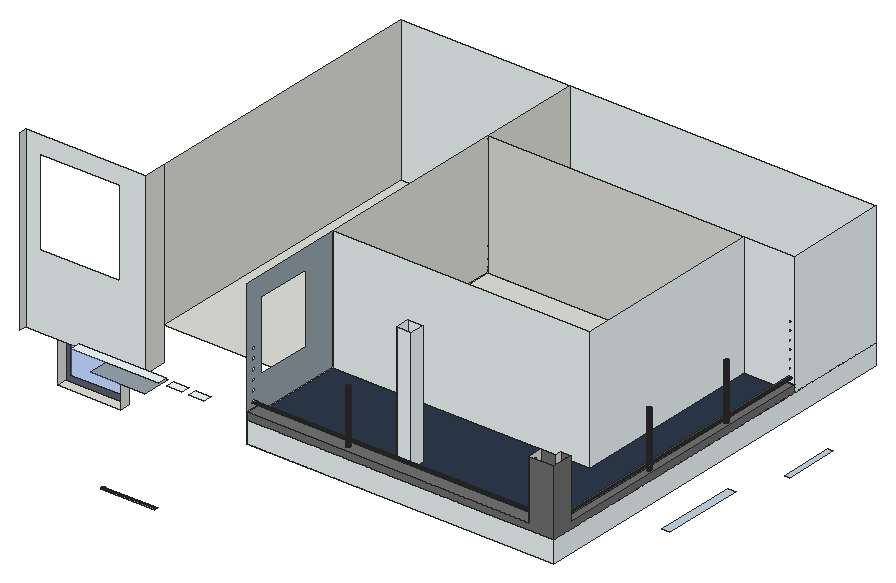
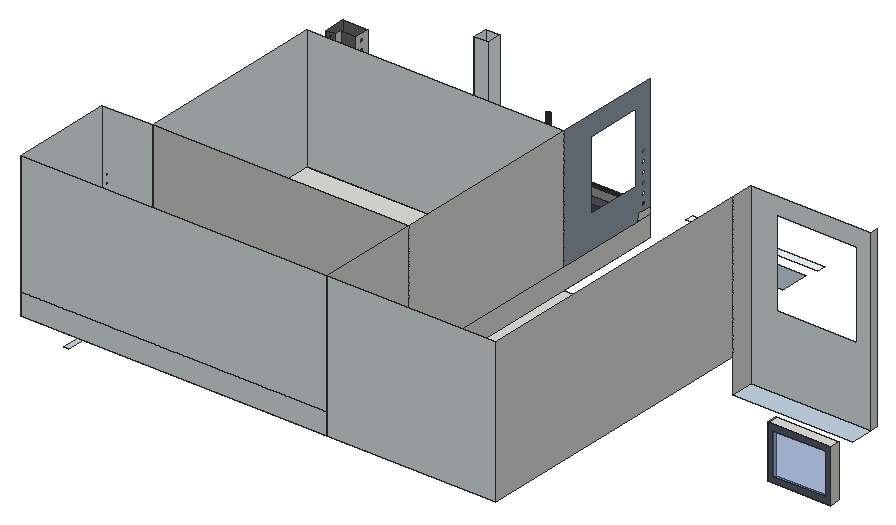
# SketchUp Ruby script. Lengths in inches.
U = 1.inch
M = Sketchup.active_model
def pt(a) = Geom::Point3d.new(a.map { |v| v * U })
def face(e, loops, mat)
  f = e.add_face(loops[0].map { |a| pt(a) })
  loops[1..].each { |l| e.add_face(l.map { |a| pt(a) }).erase! }
  f.material = f.back_material = mat if mat
  f
end
# faces: each face lists its corners as indices into pts; further lists are holes
def faces(e, pts, list, mat = nil) = list.each { |f| face(e, (f[0].is_a?(Array) ? f : [f]).map { |l| l.map { |i| pts[i] } }, mat) }
# xy, xz, yz: faces in a plane at the given z, y or x. An outline is a flat list of corners, or four numbers for a rectangle; further outlines are holes
def ring(l) = l.size == 4 ? [[l[0], l[1]], [l[2], l[1]], [l[2], l[3]], [l[0], l[3]]] : l.each_slice(2).to_a
def flat(e, list, mat, &to3) = list.each { |f| face(e, (f[0].is_a?(Array) ? f : [f]).map { |l| ring(l).map { |u, v| to3.(u, v) } }, mat) }
def xy(e, z, list, mat = nil) = flat(e, list, mat) { |x, y| [x, y, z] }
def xz(e, y, list, mat = nil) = flat(e, list, mat) { |x, z| [x, y, z] }
def yz(e, x, list, mat = nil) = flat(e, list, mat) { |y, z| [x, y, z] }
def lines(e, pts, list) = list.each { |a, b| e.add_line(pt(pts[a]), pt(pts[b])) }
# prism: a flat outline (further loops are holes) pulled along v
def prism(e, loops, v, mat = nil)
  f = face(e, loops, mat); d = Geom::Vector3d.new(v.map { |x| x * U })
  f.pushpull(f.normal.samedirection?(d) ? d.length : -d.length)
end
def box(e, o, s, mat = nil) = prism(e, [[o, [o[0] + s[0], o[1], o[2]], [o[0] + s[0], o[1] + s[1], o[2]], [o[0], o[1] + s[1], o[2]]]], [0, 0, s[2]], mat)
def at(x, y, z, deg = 0) = Geom::Transformation.translation(pt([x, y, z])) * Geom::Transformation.rotation(ORIGIN, Z_AXIS, deg.degrees)
def axes(o, x, y, z) = Geom::Transformation.new([*x, 0, *y, 0, *z, 0, *pt(o).to_a, 1])
def part(name) = M.definitions.add(name)
# library, detail: a bought-in or finely detailed component or shape, given as its bounding box
def library(name, o, s) = part(name).tap { |d| box(d.entities, o, s) }
def detail(e, o, s) = box(e.add_group.entities, o, s)
def put(e, d, t, mat = nil) = e.add_instance(d, t).tap { |i| i.material = mat if mat }
def group(e, t, mat = nil) = e.add_group.tap { |g| g.transformation = t; g.material = mat if mat }.entities
root = M.entities
M.materials.add("[Color M03]").color = [170, 170, 170]
M.materials.add("[Color M04]").color = [142, 142, 142]
M.materials.add("[Color M05]").color = [114, 114, 114]
M.materials.add("[Formica Graystone]").color = [229, 224, 207]
M.materials.add("[Formica Laminate Dark]").color = [95, 101, 114]
M.materials.add("[Leather Blue]").color = [45, 57, 74]
M.materials.add("[Terrazzo Light Blue]").color = [151, 165, 175]
M.materials.add("[Terrazzo Light Blue]1").color = [196, 214, 227]
M.materials.add("[Translucent Glass Blue]").color = [100, 149, 237]
M.materials["[Translucent Glass Blue]"].alpha = 0.5
M.materials.add("[White Subway Tile]").color = [243, 252, 253]
xy(root,1457.66,[[601.67,1239.01,858.23,1281.39]])
xy(root,1615.93,[[2949.18,2002.64,2968.68,2223.02]],"[Terrazzo Light Blue]1")
xy(root,1670.72,[[601.67,1239.01,858.23,1281.39]])
xy(root,1686.6,[[2936.43,1390.76,2968.68,1726.13]],"[Terrazzo Light Blue]1")
xy(root,1690.66,[[547.35,1146.14,1034.97,1239.01]],"[Terrazzo Light Blue]1")
xy(root,1828.125,[[2898.76,803.71,2968.68,1239.01],[1034.97,1239.01,1720.33,2442.87],[1720.33,1239.01,2968.68,2442.87]])
xy(root,1828.125,[[1720.33,803.71,2898.76,1239.01]],"[Terrazzo Light Blue]1")
xy(root,1889.95,[[1113.04,767.89,1334.04,884.27]],"[Terrazzo Light Blue]")
xy(root,1914,[[1720.33,803.71,1720.33,862.88,2929.99,862.88,2929.99,2026.57,2968.68,2026.57,2968.68,803.71],[2267.4,882.09,2324.97,939.65],[1720.33,1239.01,2764.79,2026.57],[1720.33,2026.57,2968.68,2442.87]])
xy(root,1914,[[[1720.33,862.88,2929.99,862.88,2929.99,2026.57,2764.79,2026.57,2764.79,1239.01,1720.33,1239.01],[2267.4,882.09,2324.97,939.65]]],"[Leather Blue]")
xy(root,1942.6875,[[2109.83,824.72,2107.72,824.99,2105.74,825.8125,2104.04,827.11,2102.74,828.81,2101.93,830.78,2101.65,832.9,2101.93,835.02,2102.74,837,2104.04,838.69,2105.74,839.99,2107.72,840.8125,2109.83,841.09,2111.95,840.8125,2113.93,839.99,2115.625,838.69,2116.92,837,2117.74,835.02,2118.02,832.9,2117.74,830.78,2116.92,828.81,2115.625,827.11,2113.93,825.8125,2111.95,824.99],[2949.99,1302.69,2947.9375,1302.96,2946.02,1303.75,2944.38,1305.01,2943.12,1306.66,2942.32,1308.57,2942.05,1310.63,2942.32,1312.68,2943.12,1314.6,2944.38,1316.24,2946.02,1317.5,2947.9375,1318.29,2949.99,1318.56,2952.05,1318.29,2953.96,1317.5,2955.6,1316.24,2956.87,1314.6,2957.66,1312.68,2957.93,1310.63,2957.66,1308.57,2956.87,1306.66,2955.6,1305.01,2953.96,1303.75,2952.05,1302.96],[2949.99,1696.19,2947.9375,1696.46,2946.02,1697.25,2944.38,1698.51,2943.12,1700.16,2942.32,1702.07,2942.05,1704.13,2942.32,1706.18,2943.12,1708.1,2944.38,1709.74,2946.02,1711,2947.9375,1711.79,2949.99,1712.06,2952.05,1711.79,2953.96,1711,2955.6,1709.74,2956.87,1708.1,2957.66,1706.18,2957.93,1704.13,2957.66,1702.07,2956.87,1700.16,2955.6,1698.51,2953.96,1697.25,2952.05,1696.46]])
xy(root,1942.6875,[[[1720.33,803.71,2867.16,862.88],[2109.83,824.72,2107.72,824.99,2105.74,825.8125,2104.04,827.11,2102.74,828.81,2101.93,830.78,2101.65,832.9,2101.93,835.02,2102.74,837,2104.04,838.69,2105.74,839.99,2107.72,840.8125,2109.83,841.09,2111.95,840.8125,2113.93,839.99,2115.625,838.69,2116.92,837,2117.74,835.02,2118.02,832.9,2117.74,830.78,2116.92,828.81,2115.625,827.11,2113.93,825.8125,2111.95,824.99]],[[2929.99,888.17,2968.68,2026.57],[2949.99,1302.69,2947.9375,1302.96,2946.02,1303.75,2944.38,1305.01,2943.12,1306.66,2942.32,1308.57,2942.05,1310.63,2942.32,1312.68,2943.12,1314.6,2944.38,1316.24,2946.02,1317.5,2947.9375,1318.29,2949.99,1318.56,2952.05,1318.29,2953.96,1317.5,2955.6,1316.24,2956.87,1314.6,2957.66,1312.68,2957.93,1310.63,2957.66,1308.57,2956.87,1306.66,2955.6,1305.01,2953.96,1303.75,2952.05,1302.96],[2949.99,1696.19,2947.9375,1696.46,2946.02,1697.25,2944.38,1698.51,2943.12,1700.16,2942.32,1702.07,2942.05,1704.13,2942.32,1706.18,2943.12,1708.1,2944.38,1709.74,2946.02,1711,2947.9375,1711.79,2949.99,1712.06,2952.05,1711.79,2953.96,1711,2955.6,1709.74,2956.87,1708.1,2957.66,1706.18,2957.93,1704.13,2957.66,1702.07,2956.87,1700.16,2955.6,1698.51,2953.96,1697.25,2952.05,1696.46]]],"[Color M05]")
xy(root,1947.36,[[1421.94,767.89,1482.63,803.71],[1511.44,767.89,1572.13,803.71]],"[White Subway Tile]")
xy(root,1949.53,[[1034.97,767.89,1389.66,803.71]],"[White Subway Tile]")
xz(root,803.71,[[1720.33,1914,2968.68,1914,2968.68,2183.75,2867.16,2183.75,2867.16,1942.6875,1720.33,1942.6875]],"[Color M05]")
xz(root,803.71,[[1720.33,1828.125,2968.68,1914]],"[White Subway Tile]")
xz(root,862.88,[[1720.33,1914,1720.33,1942.6875,2867.16,1942.6875,2867.16,2183.75,2929.99,2183.75,2929.99,1914]],"[Color M05]")
xz(root,882.09,[[2267.4,1914,2324.97,2410.6875]],"[White Subway Tile]")
xz(root,888.17,[[2950.45,1956.78,2952.01,1956.99,2953.45,1957.59,2954.7,1958.54,2955.65,1959.78,2956.25,1961.23,2956.45,1962.78,2956.25,1964.34,2955.65,1965.78,2954.7,1967.03,2953.45,1967.98,2952.01,1968.58,2950.45,1968.78,2948.9,1968.58,2947.45,1967.98,2946.21,1967.03,2945.26,1965.78,2944.66,1964.34,2944.45,1962.78,2944.66,1961.23,2945.26,1959.78,2946.21,1958.54,2947.45,1957.59,2948.9,1956.99]])
xz(root,888.17,[[[2929.99,1942.6875,2968.68,2183.75],[2950.45,1956.78,2952.01,1956.99,2953.45,1957.59,2954.7,1958.54,2955.65,1959.78,2956.25,1961.23,2956.45,1962.78,2956.25,1964.34,2955.65,1965.78,2954.7,1967.03,2953.45,1967.98,2952.01,1968.58,2950.45,1968.78,2948.9,1968.58,2947.45,1967.98,2946.21,1967.03,2945.26,1965.78,2944.66,1964.34,2944.45,1962.78,2944.66,1961.23,2945.26,1959.78,2946.21,1958.54,2947.45,1957.59,2948.9,1956.99],[2950.45,2128.53,2952.01,2128.74,2953.45,2129.34,2954.7,2130.29,2955.65,2131.53,2956.25,2132.98,2956.45,2134.53,2956.25,2136.09,2955.65,2137.53,2954.7,2138.78,2953.45,2139.73,2952.01,2140.33,2950.45,2140.53,2948.9,2140.33,2947.45,2139.73,2946.21,2138.78,2945.26,2137.53,2944.66,2136.09,2944.45,2134.53,2944.66,2132.98,2945.26,2131.53,2946.21,2130.29,2947.45,2129.34,2948.9,2128.74],[2950.45,1989.28,2952.01,1989.49,2953.45,1990.09,2954.7,1991.04,2955.65,1992.28,2956.25,1993.73,2956.45,1995.28,2956.25,1996.84,2955.65,1998.28,2954.7,1999.53,2953.45,2000.48,2952.01,2001.08,2950.45,2001.28,2948.9,2001.08,2947.45,2000.48,2946.21,1999.53,2945.26,1998.28,2944.66,1996.84,2944.45,1995.28,2944.66,1993.73,2945.26,1992.28,2946.21,1991.04,2947.45,1990.09,2948.9,1989.49],[2950.45,2090.97,2952.01,2091.18,2953.45,2091.77,2954.7,2092.73,2955.65,2093.97,2956.25,2095.42,2956.45,2096.97,2956.25,2098.52,2955.65,2099.97,2954.7,2101.21,2953.45,2102.17,2952.01,2102.77,2950.45,2102.97,2948.9,2102.77,2947.45,2102.17,2946.21,2101.21,2945.26,2099.97,2944.66,2098.52,2944.45,2096.97,2944.66,2095.42,2945.26,2093.97,2946.21,2092.73,2947.45,2091.77,2948.9,2091.18],[2950.45,2021.91,2952.01,2022.11,2953.45,2022.71,2954.7,2023.67,2955.65,2024.91,2956.25,2026.36,2956.45,2027.91,2956.25,2029.46,2955.65,2030.91,2954.7,2032.15,2953.45,2033.1,2952.01,2033.7,2950.45,2033.91,2948.9,2033.7,2947.45,2033.1,2946.21,2032.15,2945.26,2030.91,2944.66,2029.46,2944.45,2027.91,2944.66,2026.36,2945.26,2024.91,2946.21,2023.67,2947.45,2022.71,2948.9,2022.11],[2950.45,2059.47,2952.01,2059.68,2953.45,2060.27,2954.7,2061.23,2955.65,2062.47,2956.25,2063.92,2956.45,2065.47,2956.25,2067.02,2955.65,2068.47,2954.7,2069.71,2953.45,2070.67,2952.01,2071.27,2950.45,2071.47,2948.9,2071.27,2947.45,2070.67,2946.21,2069.71,2945.26,2068.47,2944.66,2067.02,2944.45,2065.47,2944.66,2063.92,2945.26,2062.47,2946.21,2061.23,2947.45,2060.27,2948.9,2059.68],[2950.45,2161.72,2952.01,2161.93,2953.45,2162.52,2954.7,2163.48,2955.65,2164.72,2956.25,2166.17,2956.45,2167.72,2956.25,2169.27,2955.65,2170.72,2954.7,2171.96,2953.45,2172.92,2952.01,2173.52,2950.45,2173.72,2948.9,2173.52,2947.45,2172.92,2946.21,2171.96,2945.26,2170.72,2944.66,2169.27,2944.45,2167.72,2944.66,2166.17,2945.26,2164.72,2946.21,2163.48,2947.45,2162.52,2948.9,2161.93]]],"[Color M05]")
xz(root,939.65,[[2267.4,1914,2324.97,2410.6875]],"[White Subway Tile]")
xz(root,1146.14,[[[547.35,1690.66,1034.97,2410.6875],[605.8,1990.62,928.48,2340.5]]],"[White Subway Tile]")
xz(root,1239.01,[[1925.5625,1566.2,2014.55,1621.2],[2058.375,1566.2,2147.37,1621.2]],"[Formica Graystone]")
xz(root,1239.01,[[1720.33,1914,2764.79,2410.6875]],"[White Subway Tile]")
xz(root,1281.39,[[[601.67,1457.66,858.23,1670.72],[623.88,1479.87,836.02,1648.51]]],"[Formica Laminate Dark]")
xz(root,1281.39,[[623.88,1479.87,836.02,1648.51]],"[Translucent Glass Blue]")
xz(root,2026.57,[[1720.33,1914,2764.79,2410.6875],[2929.99,1914,2968.68,1942.6875]])
xz(root,2026.57,[[[2764.79,1914,2929.99,1914,2929.99,1942.6875,2968.68,1942.6875,2968.68,2410.6875,2764.79,2410.6875],[2950.45,2161.72,2948.9,2161.93,2947.45,2162.52,2946.21,2163.48,2945.26,2164.72,2944.66,2166.17,2944.45,2167.72,2944.66,2169.27,2945.26,2170.72,2946.21,2171.96,2947.45,2172.92,2948.9,2173.52,2950.45,2173.72,2952.01,2173.52,2953.45,2172.92,2954.7,2171.96,2955.65,2170.72,2956.25,2169.27,2956.45,2167.72,2956.25,2166.17,2955.65,2164.72,2954.7,2163.48,2953.45,2162.52,2952.01,2161.93],[2950.45,2128.53,2948.9,2128.74,2947.45,2129.34,2946.21,2130.29,2945.26,2131.53,2944.66,2132.98,2944.45,2134.53,2944.66,2136.09,2945.26,2137.53,2946.21,2138.78,2947.45,2139.73,2948.9,2140.33,2950.45,2140.53,2952.01,2140.33,2953.45,2139.73,2954.7,2138.78,2955.65,2137.53,2956.25,2136.09,2956.45,2134.53,2956.25,2132.98,2955.65,2131.53,2954.7,2130.29,2953.45,2129.34,2952.01,2128.74],[2950.45,2090.97,2948.9,2091.18,2947.45,2091.77,2946.21,2092.73,2945.26,2093.97,2944.66,2095.42,2944.45,2096.97,2944.66,2098.52,2945.26,2099.97,2946.21,2101.21,2947.45,2102.17,2948.9,2102.77,2950.45,2102.97,2952.01,2102.77,2953.45,2102.17,2954.7,2101.21,2955.65,2099.97,2956.25,2098.52,2956.45,2096.97,2956.25,2095.42,2955.65,2093.97,2954.7,2092.73,2953.45,2091.77,2952.01,2091.18],[2950.45,2059.47,2948.9,2059.68,2947.45,2060.27,2946.21,2061.23,2945.26,2062.47,2944.66,2063.92,2944.45,2065.47,2944.66,2067.02,2945.26,2068.47,2946.21,2069.71,2947.45,2070.67,2948.9,2071.27,2950.45,2071.47,2952.01,2071.27,2953.45,2070.67,2954.7,2069.71,2955.65,2068.47,2956.25,2067.02,2956.45,2065.47,2956.25,2063.92,2955.65,2062.47,2954.7,2061.23,2953.45,2060.27,2952.01,2059.68],[2950.45,2021.91,2948.9,2022.11,2947.45,2022.71,2946.21,2023.67,2945.26,2024.91,2944.66,2026.36,2944.45,2027.91,2944.66,2029.46,2945.26,2030.91,2946.21,2032.15,2947.45,2033.1,2948.9,2033.7,2950.45,2033.91,2952.01,2033.7,2953.45,2033.1,2954.7,2032.15,2955.65,2030.91,2956.25,2029.46,2956.45,2027.91,2956.25,2026.36,2955.65,2024.91,2954.7,2023.67,2953.45,2022.71,2952.01,2022.11],[2950.45,1989.28,2948.9,1989.49,2947.45,1990.09,2946.21,1991.04,2945.26,1992.28,2944.66,1993.73,2944.45,1995.28,2944.66,1996.84,2945.26,1998.28,2946.21,1999.53,2947.45,2000.48,2948.9,2001.08,2950.45,2001.28,2952.01,2001.08,2953.45,2000.48,2954.7,1999.53,2955.65,1998.28,2956.25,1996.84,2956.45,1995.28,2956.25,1993.73,2955.65,1992.28,2954.7,1991.04,2953.45,1990.09,2952.01,1989.49],[2950.45,1956.78,2948.9,1956.99,2947.45,1957.59,2946.21,1958.54,2945.26,1959.78,2944.66,1961.23,2944.45,1962.78,2944.66,1964.34,2945.26,1965.78,2946.21,1967.03,2947.45,1967.98,2948.9,1968.58,2950.45,1968.78,2952.01,1968.58,2953.45,1967.98,2954.7,1967.03,2955.65,1965.78,2956.25,1964.34,2956.45,1962.78,2956.25,1961.23,2955.65,1959.78,2954.7,1958.54,2953.45,1957.59,2952.01,1956.99]]],"[White Subway Tile]")
xz(root,2442.87,[[1034.97,1828.125,1720.33,2410.6875],[1720.33,1828.125,2968.68,1914],[1720.33,1914,2968.68,2410.6875]],"[White Subway Tile]")
yz(root,547.35,[[1118.14,1690.66,1146.14,2410.6875]])
yz(root,601.67,[[1239.01,1457.66,1281.39,1670.72]])
yz(root,858.23,[[1239.01,1457.66,1281.39,1670.72]])
yz(root,1034.97,[[1146.14,1690.66,1239.01,2410.6875],[1239.01,1828.125,2442.87,2410.6875]])
yz(root,1720.33,[[803.71,1828.125,2442.87,1914],[803.71,1914,862.88,1942.6875],[1239.01,1914,2026.57,2410.6875],[2026.57,1914,2442.87,2410.6875]])
yz(root,1720.33,[[[862.88,1914,1239.01,1914,1239.01,2410.6875,803.71,2410.6875,803.71,1942.6875,862.88,1942.6875],[876.99,2047.68,1103.3,2330.11],[836.16,2153.1,834.125,2153.37,832.22,2154.16,830.59,2155.41,829.34,2157.04,828.55,2158.9375,828.29,2160.98,828.55,2163.02,829.34,2164.91,830.59,2166.55,832.22,2167.8,834.125,2168.58,836.16,2168.85,838.2,2168.58,840.1,2167.8,841.73,2166.55,842.98,2164.91,843.77,2163.02,844.04,2160.98,843.77,2158.9375,842.98,2157.04,841.73,2155.41,840.1,2154.16,838.2,2153.37],[836.16,2115.79,834.125,2116.06,832.22,2116.84,830.59,2118.1,829.34,2119.73,828.55,2121.625,828.29,2123.66,828.55,2125.7,829.34,2127.6,830.59,2129.23,832.22,2130.48,834.125,2131.27,836.16,2131.54,838.2,2131.27,840.1,2130.48,841.73,2129.23,842.98,2127.6,843.77,2125.7,844.04,2123.66,843.77,2121.625,842.98,2119.73,841.73,2118.1,840.1,2116.84,838.2,2116.06],[836.16,2075.23,834.125,2075.5,832.22,2076.28,830.59,2077.53,829.34,2079.16,828.55,2081.0625,828.29,2083.1,828.55,2085.14,829.34,2087.04,830.59,2088.67,832.22,2089.92,834.125,2090.71,836.16,2090.98,838.2,2090.71,840.1,2089.92,841.73,2088.67,842.98,2087.04,843.77,2085.14,844.04,2083.1,843.77,2081.0625,842.98,2079.16,841.73,2077.53,840.1,2076.28,838.2,2075.5],[836.16,2037.54,834.125,2037.81,832.22,2038.59,830.59,2039.85,829.34,2041.48,828.55,2043.375,828.29,2045.41,828.55,2047.45,829.34,2049.35,830.59,2050.98,832.22,2052.23,834.125,2053.02,836.16,2053.29,838.2,2053.02,840.1,2052.23,841.73,2050.98,842.98,2049.35,843.77,2047.45,844.04,2045.41,843.77,2043.375,842.98,2041.48,841.73,2039.85,840.1,2038.59,838.2,2037.81],[836.16,1998.66,834.125,1998.93,832.22,1999.72,830.59,2000.97,829.34,2002.6,828.55,2004.5,828.29,2006.54,828.55,2008.58,829.34,2010.48,830.59,2012.11,832.22,2013.36,834.125,2014.15,836.16,2014.41,838.2,2014.15,840.1,2013.36,841.73,2012.11,842.98,2010.48,843.77,2008.58,844.04,2006.54,843.77,2004.5,842.98,2002.6,841.73,2000.97,840.1,1999.72,838.2,1998.93],[836.16,1961.35,834.125,1961.62,832.22,1962.41,830.59,1963.66,829.34,1965.29,828.55,1967.1875,828.29,1969.23,828.55,1971.27,829.34,1973.16,830.59,1974.8,832.22,1976.05,834.125,1976.83,836.16,1977.1,838.2,1976.83,840.1,1976.05,841.73,1974.8,842.98,1973.16,843.77,1971.27,844.04,1969.23,843.77,1967.1875,842.98,1965.29,841.73,1963.66,840.1,1962.41,838.2,1961.62]]],"[Terrazzo Light Blue]")
yz(root,2267.4,[[882.09,1914,939.65,2410.6875]],"[White Subway Tile]")
yz(root,2324.97,[[882.09,1914,939.65,2410.6875]],"[White Subway Tile]")
yz(root,2764.79,[[1239.01,1914,2026.57,2410.6875]],"[White Subway Tile]")
yz(root,2867.16,[[[803.71,1942.6875,862.88,2183.75],[836.16,1961.35,838.2,1961.62,840.1,1962.41,841.73,1963.66,842.98,1965.29,843.77,1967.1875,844.04,1969.23,843.77,1971.27,842.98,1973.16,841.73,1974.8,840.1,1976.05,838.2,1976.83,836.16,1977.1,834.125,1976.83,832.22,1976.05,830.59,1974.8,829.34,1973.16,828.55,1971.27,828.29,1969.23,828.55,1967.1875,829.34,1965.29,830.59,1963.66,832.22,1962.41,834.125,1961.62],[836.16,2115.79,838.2,2116.06,840.1,2116.84,841.73,2118.1,842.98,2119.73,843.77,2121.625,844.04,2123.66,843.77,2125.7,842.98,2127.6,841.73,2129.23,840.1,2130.48,838.2,2131.27,836.16,2131.54,834.125,2131.27,832.22,2130.48,830.59,2129.23,829.34,2127.6,828.55,2125.7,828.29,2123.66,828.55,2121.625,829.34,2119.73,830.59,2118.1,832.22,2116.84,834.125,2116.06],[836.16,1998.66,838.2,1998.93,840.1,1999.72,841.73,2000.97,842.98,2002.6,843.77,2004.5,844.04,2006.54,843.77,2008.58,842.98,2010.48,841.73,2012.11,840.1,2013.36,838.2,2014.15,836.16,2014.41,834.125,2014.15,832.22,2013.36,830.59,2012.11,829.34,2010.48,828.55,2008.58,828.29,2006.54,828.55,2004.5,829.34,2002.6,830.59,2000.97,832.22,1999.72,834.125,1998.93],[836.16,2075.23,838.2,2075.5,840.1,2076.28,841.73,2077.53,842.98,2079.16,843.77,2081.0625,844.04,2083.1,843.77,2085.14,842.98,2087.04,841.73,2088.67,840.1,2089.92,838.2,2090.71,836.16,2090.98,834.125,2090.71,832.22,2089.92,830.59,2088.67,829.34,2087.04,828.55,2085.14,828.29,2083.1,828.55,2081.0625,829.34,2079.16,830.59,2077.53,832.22,2076.28,834.125,2075.5],[836.16,2037.54,838.2,2037.81,840.1,2038.59,841.73,2039.85,842.98,2041.48,843.77,2043.375,844.04,2045.41,843.77,2047.45,842.98,2049.35,841.73,2050.98,840.1,2052.23,838.2,2053.02,836.16,2053.29,834.125,2053.02,832.22,2052.23,830.59,2050.98,829.34,2049.35,828.55,2047.45,828.29,2045.41,828.55,2043.375,829.34,2041.48,830.59,2039.85,832.22,2038.59,834.125,2037.81],[836.16,2153.1,838.2,2153.37,840.1,2154.16,841.73,2155.41,842.98,2157.04,843.77,2158.9375,844.04,2160.98,843.77,2163.02,842.98,2164.91,841.73,2166.55,840.1,2167.8,838.2,2168.58,836.16,2168.85,834.125,2168.58,832.22,2167.8,830.59,2166.55,829.34,2164.91,828.55,2163.02,828.29,2160.98,828.55,2158.9375,829.34,2157.04,830.59,2155.41,832.22,2154.16,834.125,2153.37]],[836.16,1961.35,838.2,1961.62,840.1,1962.41,841.73,1963.66,842.98,1965.29,843.77,1967.1875,844.04,1969.23,843.77,1971.27,842.98,1973.16,841.73,1974.8,840.1,1976.05,838.2,1976.83,836.16,1977.1,834.125,1976.83,832.22,1976.05,830.59,1974.8,829.34,1973.16,828.55,1971.27,828.29,1969.23,828.55,1967.1875,829.34,1965.29,830.59,1963.66,832.22,1962.41,834.125,1961.62]])
yz(root,2929.99,[[862.88,1914,862.88,2183.75,888.17,2183.75,888.17,1942.6875,2026.57,1942.6875,2026.57,1914]])
yz(root,2968.68,[[803.71,1914,2026.57,1914,2026.57,1942.6875,888.17,1942.6875,888.17,2183.75,803.71,2183.75]],"[Color M05]")
yz(root,2968.68,[[803.71,1828.125,2442.87,1914],[2026.57,1914,2442.87,2410.6875]],"[White Subway Tile]")
p = [[1334.04,819.75,1444.12],[1334.04,821.6,1445.54],[1113.04,821.6,1445.54],[1113.04,819.75,1444.12],[1334.04,830.54,1445.54],[1334.04,832.39,1444.12],
  [1113.04,832.39,1444.12],[1113.04,830.54,1445.54],[1334.04,823.76,1446.43],[1113.04,823.76,1446.43],[1334.04,828.38,1446.43],[1113.04,828.38,1446.43],
  [1334.04,826.07,1446.73],[1113.04,826.07,1446.73],[2107.72,824.99,1942.6875],[2109.83,824.72,1942.6875],[2109.83,824.72,2160.625],[2107.72,824.99,2160.625],
  [2111.95,824.99,1942.6875],[2111.95,824.99,2160.625],[2105.74,825.8125,1942.6875],[2105.74,825.8125,2160.625],[2113.93,825.8125,1942.6875],[2113.93,825.8125,2160.625],
  [2104.04,827.11,1942.6875],[2104.04,827.11,2160.625],[2115.625,827.11,1942.6875],[2115.625,827.11,2160.625],[2102.74,828.81,1942.6875],[2102.74,828.81,2160.625],
  [2116.92,828.81,1942.6875],[2116.92,828.81,2160.625],[2101.93,830.78,1942.6875],[2101.93,830.78,2160.625],[2117.74,830.78,1942.6875],[2117.74,830.78,2160.625],
  [2101.65,832.9,1942.6875],[2101.65,832.9,2160.625],[2118.02,832.9,1942.6875],[2118.02,832.9,2160.625],[2101.93,835.02,1942.6875],[2101.93,835.02,2160.625],
  [2117.74,835.02,1942.6875],[2117.74,835.02,2160.625],[2102.74,837,1942.6875],[2102.74,837,2160.625],[2116.92,837,1942.6875],[2116.92,837,2160.625],
  [2104.04,838.69,1942.6875],[2104.04,838.69,2160.625],[2115.625,838.69,1942.6875],[2115.625,838.69,2160.625],[2105.74,839.99,1942.6875],[2105.74,839.99,2160.625],
  [2113.93,839.99,1942.6875],[2113.93,839.99,2160.625],[2107.72,840.8125,1942.6875],[2107.72,840.8125,2160.625],[2111.95,840.8125,1942.6875],[2111.95,840.8125,2160.625],
  [2109.83,841.09,1942.6875],[2109.83,841.09,2160.625],[2947.9375,1302.96,1942.6875],[2949.99,1302.69,1942.6875],[2949.99,1302.69,2167.625],[2947.9375,1302.96,2167.625],
  [2952.05,1302.96,1942.6875],[2952.05,1302.96,2167.625],[2946.02,1303.75,1942.6875],[2946.02,1303.75,2167.625],[2953.96,1303.75,1942.6875],[2953.96,1303.75,2167.625],
  [2944.38,1305.01,1942.6875],[2944.38,1305.01,2167.625],[2955.6,1305.01,1942.6875],[2955.6,1305.01,2167.625],[2943.12,1306.66,1942.6875],[2943.12,1306.66,2167.625],
  [2956.87,1306.66,1942.6875],[2956.87,1306.66,2167.625],[2942.32,1308.57,1942.6875],[2942.32,1308.57,2167.625],[2957.66,1308.57,1942.6875],[2957.66,1308.57,2167.625],
  [2942.05,1310.63,1942.6875],[2942.05,1310.63,2167.625],[2957.93,1310.63,1942.6875],[2957.93,1310.63,2167.625],[2942.32,1312.68,1942.6875],[2942.32,1312.68,2167.625],
  [2957.66,1312.68,1942.6875],[2957.66,1312.68,2167.625],[2943.12,1314.6,1942.6875],[2943.12,1314.6,2167.625],[2956.87,1314.6,1942.6875],[2956.87,1314.6,2167.625],
  [2944.38,1316.24,1942.6875],[2944.38,1316.24,2167.625],[2955.6,1316.24,1942.6875],[2955.6,1316.24,2167.625],[2946.02,1317.5,1942.6875],[2946.02,1317.5,2167.625],
  [2953.96,1317.5,1942.6875],[2953.96,1317.5,2167.625],[2947.9375,1318.29,1942.6875],[2947.9375,1318.29,2167.625],[2952.05,1318.29,1942.6875],[2952.05,1318.29,2167.625],
  [2949.99,1318.56,1942.6875],[2949.99,1318.56,2167.625],[2947.9375,1696.46,1942.6875],[2949.99,1696.19,1942.6875],[2949.99,1696.19,2167.3125],[2947.9375,1696.46,2167.3125],
  [2952.05,1696.46,1942.6875],[2952.05,1696.46,2167.3125],[2946.02,1697.25,1942.6875],[2946.02,1697.25,2167.3125],[2953.96,1697.25,1942.6875],[2953.96,1697.25,2167.3125],
  [2944.38,1698.51,1942.6875],[2944.38,1698.51,2167.3125],[2955.6,1698.51,1942.6875],[2955.6,1698.51,2167.3125],[2943.12,1700.16,1942.6875],[2943.12,1700.16,2167.3125],
  [2956.87,1700.16,1942.6875],[2956.87,1700.16,2167.3125],[2942.32,1702.07,1942.6875],[2942.32,1702.07,2167.3125],[2957.66,1702.07,1942.6875],[2957.66,1702.07,2167.3125],
  [2942.05,1704.13,1942.6875],[2942.05,1704.13,2167.3125],[2957.93,1704.13,1942.6875],[2957.93,1704.13,2167.3125],[2942.32,1706.18,1942.6875],[2942.32,1706.18,2167.3125],
  [2957.66,1706.18,1942.6875],[2957.66,1706.18,2167.3125],[2943.12,1708.1,1942.6875],[2943.12,1708.1,2167.3125],[2956.87,1708.1,1942.6875],[2956.87,1708.1,2167.3125],
  [2944.38,1709.74,1942.6875],[2944.38,1709.74,2167.3125],[2955.6,1709.74,1942.6875],[2955.6,1709.74,2167.3125],[2946.02,1711,1942.6875],[2946.02,1711,2167.3125],
  [2953.96,1711,1942.6875],[2953.96,1711,2167.3125],[2947.9375,1711.79,1942.6875],[2947.9375,1711.79,2167.3125],[2952.05,1711.79,1942.6875],[2952.05,1711.79,2167.3125],
  [2949.99,1712.06,1942.6875],[2949.99,1712.06,2167.3125],[2950.45,888.17,1956.78],[2948.9,888.17,1956.99],[2948.9,2026.57,1956.99],[2950.45,2026.57,1956.78],
  [2952.01,888.17,1956.99],[2952.01,2026.57,1956.99],[2947.45,888.17,1957.59],[2947.45,2026.57,1957.59],[2953.45,888.17,1957.59],[2953.45,2026.57,1957.59],
  [2946.21,888.17,1958.54],[2946.21,2026.57,1958.54],[2954.7,888.17,1958.54],[2954.7,2026.57,1958.54],[2945.26,888.17,1959.78],[2945.26,2026.57,1959.78],
  [2955.65,888.17,1959.78],[2955.65,2026.57,1959.78],[2944.66,888.17,1961.23],[2944.66,2026.57,1961.23],[2956.25,888.17,1961.23],[2956.25,2026.57,1961.23],
  [2944.45,888.17,1962.78],[2944.45,2026.57,1962.78],[2956.45,888.17,1962.78],[2956.45,2026.57,1962.78],[2867.16,836.16,1961.35],[2867.16,834.125,1961.62],
  [1720.33,834.125,1961.62],[1720.33,836.16,1961.35],[2867.16,838.2,1961.62],[1720.33,838.2,1961.62],[2867.16,832.22,1962.41],[1720.33,832.22,1962.41],
  [2867.16,840.1,1962.41],[1720.33,840.1,1962.41],[2867.16,830.59,1963.66],[1720.33,830.59,1963.66],[2867.16,841.73,1963.66],[1720.33,841.73,1963.66],
  [2944.66,888.17,1964.34],[2944.66,2026.57,1964.34],[2956.25,888.17,1964.34],[2956.25,2026.57,1964.34],[2867.16,829.34,1965.29],[1720.33,829.34,1965.29],
  [2867.16,842.98,1965.29],[1720.33,842.98,1965.29],[2945.26,888.17,1965.78],[2945.26,2026.57,1965.78],[2955.65,888.17,1965.78],[2955.65,2026.57,1965.78],
  [2867.16,828.55,1967.1875],[1720.33,828.55,1967.1875],[2867.16,843.77,1967.1875],[1720.33,843.77,1967.1875],[2946.21,888.17,1967.03],[2946.21,2026.57,1967.03],
  [2954.7,888.17,1967.03],[2954.7,2026.57,1967.03]]
faces(root,p,[[0,1,2,3],[4,5,6,7],[1,8,9,2],[10,4,7,11],[8,12,13,9],[12,10,11,13]],"[Color M03]")
faces(root,p,[[14,15,16,17],[15,18,19,16],[20,14,17,21],[18,22,23,19],[24,20,21,25],[22,26,27,23],[28,24,25,29],[26,30,31,27],
  [32,28,29,33],[30,34,35,31],[36,32,33,37],[34,38,39,35],[40,36,37,41],[38,42,43,39],[44,40,41,45],[42,46,47,43],
  [48,44,45,49],[46,50,51,47],[52,48,49,53],[50,54,55,51],[56,52,53,57],[54,58,59,55],[60,56,57,61],[58,60,61,59],
  [62,63,64,65],[63,66,67,64],[68,62,65,69],[66,70,71,67],[72,68,69,73],[70,74,75,71],[76,72,73,77],[74,78,79,75],
  [80,76,77,81],[78,82,83,79],[84,80,81,85],[82,86,87,83],[88,84,85,89],[86,90,91,87],[92,88,89,93],[90,94,95,91],
  [96,92,93,97],[94,98,99,95],[100,96,97,101],[98,102,103,99],[104,100,101,105],[102,106,107,103],[108,104,105,109],[106,108,109,107],
  [110,111,112,113],[111,114,115,112],[116,110,113,117],[114,118,119,115],[120,116,117,121],[118,122,123,119],[124,120,121,125],[122,126,127,123],
  [128,124,125,129],[126,130,131,127],[132,128,129,133],[130,134,135,131],[136,132,133,137],[134,138,139,135],[140,136,137,141],[138,142,143,139],
  [144,140,141,145],[142,146,147,143],[148,144,145,149],[146,150,151,147],[152,148,149,153],[150,154,155,151],[156,152,153,157],[154,156,157,155],
  [158,159,160,161],[162,158,161,163],[159,164,165,160],[166,162,163,167],[164,168,169,165],[170,166,167,171],[168,172,173,169],[174,170,171,175],
  [172,176,177,173],[178,174,175,179],[176,180,181,177],[182,178,179,183],[184,185,186,187],[188,184,187,189],[185,190,191,186],[192,188,189,193],
  [190,194,195,191],[196,192,193,197],[180,198,199,181],[200,182,183,201],[194,202,203,195],[204,196,197,205],[198,206,207,199],[208,200,201,209],
  [202,210,211,203],[212,204,205,213],[206,214,215,207],[216,208,209,217]],"[Color M04]")
